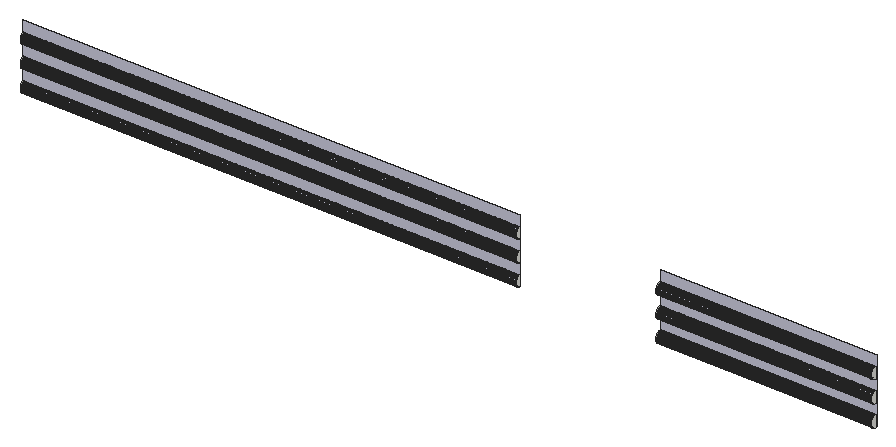
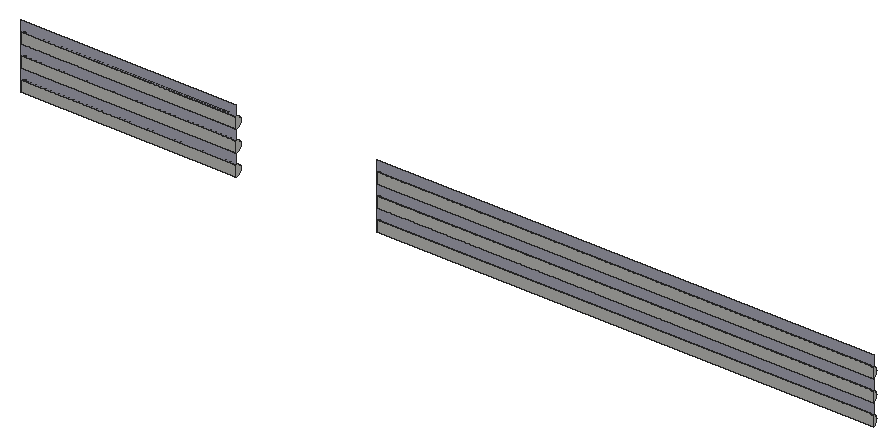
# SketchUp Ruby script. Lengths in millimetres.
U = 1.mm
M = Sketchup.active_model
def pt(a) = Geom::Point3d.new(a.map { |v| v * U })
def face(e, loops, mat)
  f = e.add_face(loops[0].map { |a| pt(a) })
  loops[1..].each { |l| e.add_face(l.map { |a| pt(a) }).erase! }
  f.material = f.back_material = mat if mat
  f
end
# faces: each face lists its corners as indices into pts; further lists are holes
def faces(e, pts, list, mat = nil) = list.each { |f| face(e, (f[0].is_a?(Array) ? f : [f]).map { |l| l.map { |i| pts[i] } }, mat) }
# xy, xz, yz: faces in a plane at the given z, y or x. An outline is a flat list of corners, or four numbers for a rectangle; further outlines are holes
def ring(l) = l.size == 4 ? [[l[0], l[1]], [l[2], l[1]], [l[2], l[3]], [l[0], l[3]]] : l.each_slice(2).to_a
def flat(e, list, mat, &to3) = list.each { |f| face(e, (f[0].is_a?(Array) ? f : [f]).map { |l| ring(l).map { |u, v| to3.(u, v) } }, mat) }
def xy(e, z, list, mat = nil) = flat(e, list, mat) { |x, y| [x, y, z] }
def xz(e, y, list, mat = nil) = flat(e, list, mat) { |x, z| [x, y, z] }
def yz(e, x, list, mat = nil) = flat(e, list, mat) { |y, z| [x, y, z] }
def lines(e, pts, list) = list.each { |a, b| e.add_line(pt(pts[a]), pt(pts[b])) }
# prism: a flat outline (further loops are holes) pulled along v
def prism(e, loops, v, mat = nil)
  f = face(e, loops, mat); d = Geom::Vector3d.new(v.map { |x| x * U })
  f.pushpull(f.normal.samedirection?(d) ? d.length : -d.length)
end
def box(e, o, s, mat = nil) = prism(e, [[o, [o[0] + s[0], o[1], o[2]], [o[0] + s[0], o[1] + s[1], o[2]], [o[0], o[1] + s[1], o[2]]]], [0, 0, s[2]], mat)
def at(x, y, z, deg = 0) = Geom::Transformation.translation(pt([x, y, z])) * Geom::Transformation.rotation(ORIGIN, Z_AXIS, deg.degrees)
def axes(o, x, y, z) = Geom::Transformation.new([*x, 0, *y, 0, *z, 0, *pt(o).to_a, 1])
def part(name) = M.definitions.add(name)
# library, detail: a bought-in or finely detailed component or shape, given as its bounding box
def library(name, o, s) = part(name).tap { |d| box(d.entities, o, s) }
def detail(e, o, s) = box(e.add_group.entities, o, s)
def put(e, d, t, mat = nil) = e.add_instance(d, t).tap { |i| i.material = mat if mat }
def group(e, t, mat = nil) = e.add_group.tap { |g| g.transformation = t; g.material = mat if mat }.entities
root = M.entities
M.materials.add("[0116_Lavender]").color = [197, 197, 214]
xz(root,16548.1,[[11038.5,11141.1,25059.3,11445.9],[29021.7,11141.1,35117.7,11445.9],[11038.5,11750.7,25059.3,12055.5],[29021.7,11750.7,35117.7,12055.5],[11038.5,12360.3,25059.3,12665.1],
  [29021.7,12360.3,35117.7,12665.1]])
xz(root,16548.1,[[11038.5,11445.9,25059.3,11750.7],[29021.7,11445.9,35117.7,11750.7],[11038.5,12055.5,25059.3,12360.3],[29021.7,12055.5,35117.7,12360.3],[11038.5,12665.1,25059.3,12969.9],
  [29021.7,12665.1,35117.7,12969.9]],"[0116_Lavender]")
yz(root,11038.5,[[16548.1,11141.1,16536.2,11146.4,16524.8,11152.7,16514,11159.8,16503.7,11167.8,16494.1,11176.6,16485.2,11186.1,16477.1,11196.2,16469.8,11207,16463.4,11218.3,16458,11230.1,16453.4,11242.3,16449.9,11254.8,16447.3,11267.6,16445.8,11280.5,16445.3,11293.5,16445.8,11306.5,16447.3,11319.4,16449.9,11332.1,16453.4,11344.6,16458,11356.8,16463.4,11368.6,16469.8,11379.9,16477.1,11390.7,16485.2,11400.9,16494.1,11410.4,16503.7,11419.2,16514,11427.1,16524.8,11434.3,16536.2,11440.5,16548.1,11445.9],[16548.1,11750.7,16536.2,11756,16524.8,11762.3,16514,11769.4,16503.7,11777.4,16494.1,11786.2,16485.2,11795.7,16477.1,11805.8,16469.8,11816.6,16463.4,11827.9,16458,11839.7,16453.4,11851.9,16449.9,11864.4,16447.3,11877.2,16445.8,11890.1,16445.3,11903.1,16445.8,11916.1,16447.3,11929,16449.9,11941.7,16453.4,11954.2,16458,11966.4,16463.4,11978.2,16469.8,11989.5,16477.1,12000.3,16485.2,12010.5,16494.1,12020,16503.7,12028.8,16514,12036.7,16524.8,12043.9,16536.2,12050.1,16548.1,12055.5],[16548.1,12360.3,16536.2,12365.6,16524.8,12371.9,16514,12379,16503.7,12387,16494.1,12395.8,16485.2,12405.3,16477.1,12415.4,16469.8,12426.2,16463.4,12437.5,16458,12449.3,16453.4,12461.5,16449.9,12474,16447.3,12486.8,16445.8,12499.7,16445.3,12512.7,16445.8,12525.7,16447.3,12538.6,16449.9,12551.3,16453.4,12563.8,16458,12576,16463.4,12587.8,16469.8,12599.1,16477.1,12609.9,16485.2,12620.1,16494.1,12629.6,16503.7,12638.4,16514,12646.3,16524.8,12653.5,16536.2,12659.7,16548.1,12665.1]])
yz(root,25059.3,[[16548.1,11141.1,16548.1,11445.9,16536.2,11440.5,16524.8,11434.3,16514,11427.1,16503.7,11419.2,16494.1,11410.4,16485.2,11400.9,16477.1,11390.7,16469.8,11379.9,16463.4,11368.6,16458,11356.8,16453.4,11344.6,16449.9,11332.1,16447.3,11319.4,16445.8,11306.5,16445.3,11293.5,16445.8,11280.5,16447.3,11267.6,16449.9,11254.8,16453.4,11242.3,16458,11230.1,16463.4,11218.3,16469.8,11207,16477.1,11196.2,16485.2,11186.1,16494.1,11176.6,16503.7,11167.8,16514,11159.8,16524.8,11152.7,16536.2,11146.4],[16548.1,11750.7,16548.1,12055.5,16536.2,12050.1,16524.8,12043.9,16514,12036.7,16503.7,12028.8,16494.1,12020,16485.2,12010.5,16477.1,12000.3,16469.8,11989.5,16463.4,11978.2,16458,11966.4,16453.4,11954.2,16449.9,11941.7,16447.3,11929,16445.8,11916.1,16445.3,11903.1,16445.8,11890.1,16447.3,11877.2,16449.9,11864.4,16453.4,11851.9,16458,11839.7,16463.4,11827.9,16469.8,11816.6,16477.1,11805.8,16485.2,11795.7,16494.1,11786.2,16503.7,11777.4,16514,11769.4,16524.8,11762.3,16536.2,11756],[16548.1,12360.3,16548.1,12665.1,16536.2,12659.7,16524.8,12653.5,16514,12646.3,16503.7,12638.4,16494.1,12629.6,16485.2,12620.1,16477.1,12609.9,16469.8,12599.1,16463.4,12587.8,16458,12576,16453.4,12563.8,16449.9,12551.3,16447.3,12538.6,16445.8,12525.7,16445.3,12512.7,16445.8,12499.7,16447.3,12486.8,16449.9,12474,16453.4,12461.5,16458,12449.3,16463.4,12437.5,16469.8,12426.2,16477.1,12415.4,16485.2,12405.3,16494.1,12395.8,16503.7,12387,16514,12379,16524.8,12371.9,16536.2,12365.6]])
yz(root,29021.7,[[16548.1,11141.1,16540.1,11141.3,16532.2,11141.9,16524.3,11143,16516.4,11144.4,16508.7,11146.3,16501,11148.5,16493.5,11151.2,16486.1,11154.3,16478.9,11157.7,16471.9,11161.5,16465.1,11165.7,16458.5,11170.2,16452.2,11175,16446.1,11180.2,16440.3,11185.7,16434.8,11191.5,16429.7,11197.6,16424.8,11203.9,16420.3,11210.5,16416.1,11217.3,16412.3,11224.3,16408.9,11231.5,16405.8,11238.9,16403.2,11246.4,16400.9,11254,16399,11261.8,16397.6,11269.6,16396.5,11277.5,16395.9,11285.5,16395.7,11293.5,16395.9,11301.5,16396.5,11309.4,16397.6,11317.3,16399,11325.2,16400.9,11332.9,16403.2,11340.6,16405.8,11348.1,16408.9,11355.5,16412.3,11362.7,16416.1,11369.7,16420.3,11376.5,16424.8,11383.1,16429.7,11389.4,16434.8,11395.5,16440.3,11401.2,16446.1,11406.7,16452.2,11411.9,16458.5,11416.8,16465.1,11421.3,16471.9,11425.5,16478.9,11429.3,16486.1,11432.7,16493.5,11435.8,16501,11438.4,16508.7,11440.7,16516.4,11442.5,16524.3,11444,16532.2,11445,16540.1,11445.7,16548.1,11445.9],[16548.1,11750.7,16540.1,11750.9,16532.2,11751.5,16524.3,11752.6,16516.4,11754,16508.7,11755.9,16501,11758.1,16493.5,11760.8,16486.1,11763.9,16478.9,11767.3,16471.9,11771.1,16465.1,11775.3,16458.5,11779.8,16452.2,11784.6,16446.1,11789.8,16440.3,11795.3,16434.8,11801.1,16429.7,11807.2,16424.8,11813.5,16420.3,11820.1,16416.1,11826.9,16412.3,11833.9,16408.9,11841.1,16405.8,11848.5,16403.2,11856,16400.9,11863.6,16399,11871.4,16397.6,11879.2,16396.5,11887.1,16395.9,11895.1,16395.7,11903.1,16395.9,11911.1,16396.5,11919,16397.6,11926.9,16399,11934.8,16400.9,11942.5,16403.2,11950.2,16405.8,11957.7,16408.9,11965.1,16412.3,11972.3,16416.1,11979.3,16420.3,11986.1,16424.8,11992.7,16429.7,11999,16434.8,12005.1,16440.3,12010.8,16446.1,12016.3,16452.2,12021.5,16458.5,12026.4,16465.1,12030.9,16471.9,12035.1,16478.9,12038.9,16486.1,12042.3,16493.5,12045.4,16501,12048,16508.7,12050.3,16516.4,12052.1,16524.3,12053.6,16532.2,12054.6,16540.1,12055.3,16548.1,12055.5],[16548.1,12360.3,16540.1,12360.5,16532.2,12361.1,16524.3,12362.2,16516.4,12363.6,16508.7,12365.5,16501,12367.7,16493.5,12370.4,16486.1,12373.5,16478.9,12376.9,16471.9,12380.7,16465.1,12384.9,16458.5,12389.4,16452.2,12394.2,16446.1,12399.4,16440.3,12404.9,16434.8,12410.7,16429.7,12416.8,16424.8,12423.1,16420.3,12429.7,16416.1,12436.5,16412.3,12443.5,16408.9,12450.7,16405.8,12458.1,16403.2,12465.6,16400.9,12473.2,16399,12481,16397.6,12488.8,16396.5,12496.7,16395.9,12504.7,16395.7,12512.7,16395.9,12520.7,16396.5,12528.6,16397.6,12536.5,16399,12544.4,16400.9,12552.1,16403.2,12559.8,16405.8,12567.3,16408.9,12574.7,16412.3,12581.9,16416.1,12588.9,16420.3,12595.7,16424.8,12602.3,16429.7,12608.6,16434.8,12614.7,16440.3,12620.4,16446.1,12625.9,16452.2,12631.1,16458.5,12636,16465.1,12640.5,16471.9,12644.7,16478.9,12648.5,16486.1,12651.9,16493.5,12655,16501,12657.6,16508.7,12659.9,16516.4,12661.7,16524.3,12663.2,16532.2,12664.2,16540.1,12664.9,16548.1,12665.1]])
yz(root,35117.7,[[16548.1,11141.1,16548.1,11445.9,16540.1,11445.7,16532.2,11445,16524.3,11444,16516.4,11442.5,16508.7,11440.7,16501,11438.4,16493.5,11435.8,16486.1,11432.7,16478.9,11429.3,16471.9,11425.5,16465.1,11421.3,16458.5,11416.8,16452.2,11411.9,16446.1,11406.7,16440.3,11401.2,16434.8,11395.5,16429.7,11389.4,16424.8,11383.1,16420.3,11376.5,16416.1,11369.7,16412.3,11362.7,16408.9,11355.5,16405.8,11348.1,16403.2,11340.6,16400.9,11332.9,16399,11325.2,16397.6,11317.3,16396.5,11309.4,16395.9,11301.5,16395.7,11293.5,16395.9,11285.5,16396.5,11277.5,16397.6,11269.6,16399,11261.8,16400.9,11254,16403.2,11246.4,16405.8,11238.9,16408.9,11231.5,16412.3,11224.3,16416.1,11217.3,16420.3,11210.5,16424.8,11203.9,16429.7,11197.6,16434.8,11191.5,16440.3,11185.7,16446.1,11180.2,16452.2,11175,16458.5,11170.2,16465.1,11165.7,16471.9,11161.5,16478.9,11157.7,16486.1,11154.3,16493.5,11151.2,16501,11148.5,16508.7,11146.3,16516.4,11144.4,16524.3,11143,16532.2,11141.9,16540.1,11141.3],[16548.1,11750.7,16548.1,12055.5,16540.1,12055.3,16532.2,12054.6,16524.3,12053.6,16516.4,12052.1,16508.7,12050.3,16501,12048,16493.5,12045.4,16486.1,12042.3,16478.9,12038.9,16471.9,12035.1,16465.1,12030.9,16458.5,12026.4,16452.2,12021.5,16446.1,12016.3,16440.3,12010.8,16434.8,12005.1,16429.7,11999,16424.8,11992.7,16420.3,11986.1,16416.1,11979.3,16412.3,11972.3,16408.9,11965.1,16405.8,11957.7,16403.2,11950.2,16400.9,11942.5,16399,11934.8,16397.6,11926.9,16396.5,11919,16395.9,11911.1,16395.7,11903.1,16395.9,11895.1,16396.5,11887.1,16397.6,11879.2,16399,11871.4,16400.9,11863.6,16403.2,11856,16405.8,11848.5,16408.9,11841.1,16412.3,11833.9,16416.1,11826.9,16420.3,11820.1,16424.8,11813.5,16429.7,11807.2,16434.8,11801.1,16440.3,11795.3,16446.1,11789.8,16452.2,11784.6,16458.5,11779.8,16465.1,11775.3,16471.9,11771.1,16478.9,11767.3,16486.1,11763.9,16493.5,11760.8,16501,11758.1,16508.7,11755.9,16516.4,11754,16524.3,11752.6,16532.2,11751.5,16540.1,11750.9],[16548.1,12360.3,16548.1,12665.1,16540.1,12664.9,16532.2,12664.2,16524.3,12663.2,16516.4,12661.7,16508.7,12659.9,16501,12657.6,16493.5,12655,16486.1,12651.9,16478.9,12648.5,16471.9,12644.7,16465.1,12640.5,16458.5,12636,16452.2,12631.1,16446.1,12625.9,16440.3,12620.4,16434.8,12614.7,16429.7,12608.6,16424.8,12602.3,16420.3,12595.7,16416.1,12588.9,16412.3,12581.9,16408.9,12574.7,16405.8,12567.3,16403.2,12559.8,16400.9,12552.1,16399,12544.4,16397.6,12536.5,16396.5,12528.6,16395.9,12520.7,16395.7,12512.7,16395.9,12504.7,16396.5,12496.7,16397.6,12488.8,16399,12481,16400.9,12473.2,16403.2,12465.6,16405.8,12458.1,16408.9,12450.7,16412.3,12443.5,16416.1,12436.5,16420.3,12429.7,16424.8,12423.1,16429.7,12416.8,16434.8,12410.7,16440.3,12404.9,16446.1,12399.4,16452.2,12394.2,16458.5,12389.4,16465.1,12384.9,16471.9,12380.7,16478.9,12376.9,16486.1,12373.5,16493.5,12370.4,16501,12367.7,16508.7,12365.5,16516.4,12363.6,16524.3,12362.2,16532.2,12361.1,16540.1,12360.5]])
p = [[25059.3,16548.1,11141.1],[25059.3,16536.2,11146.4],[11038.5,16536.2,11146.4],[11038.5,16548.1,11141.1],[35117.7,16548.1,11141.1],[35117.7,16540.1,11141.3],
  [29021.7,16540.1,11141.3],[29021.7,16548.1,11141.1],[35117.7,16532.2,11141.9],[29021.7,16532.2,11141.9],[35117.7,16524.3,11143],[29021.7,16524.3,11143],
  [35117.7,16516.4,11144.4],[29021.7,16516.4,11144.4],[35117.7,16508.7,11146.3],[29021.7,16508.7,11146.3],[35117.7,16501,11148.5],[29021.7,16501,11148.5],
  [25059.3,16524.8,11152.7],[11038.5,16524.8,11152.7],[35117.7,16493.5,11151.2],[29021.7,16493.5,11151.2],[35117.7,16486.1,11154.3],[29021.7,16486.1,11154.3],
  [25059.3,16514,11159.8],[11038.5,16514,11159.8],[35117.7,16478.9,11157.7],[29021.7,16478.9,11157.7],[35117.7,16471.9,11161.5],[29021.7,16471.9,11161.5],
  [25059.3,16503.7,11167.8],[11038.5,16503.7,11167.8],[35117.7,16465.1,11165.7],[29021.7,16465.1,11165.7],[35117.7,16458.5,11170.2],[29021.7,16458.5,11170.2],
  [25059.3,16494.1,11176.6],[11038.5,16494.1,11176.6],[35117.7,16452.2,11175],[29021.7,16452.2,11175],[35117.7,16446.1,11180.2],[29021.7,16446.1,11180.2],
  [25059.3,16485.2,11186.1],[11038.5,16485.2,11186.1],[35117.7,16440.3,11185.7],[29021.7,16440.3,11185.7],[35117.7,16434.8,11191.5],[29021.7,16434.8,11191.5],
  [25059.3,16477.1,11196.2],[11038.5,16477.1,11196.2],[35117.7,16429.7,11197.6],[29021.7,16429.7,11197.6],[25059.3,16469.8,11207],[11038.5,16469.8,11207],
  [35117.7,16424.8,11203.9],[29021.7,16424.8,11203.9],[35117.7,16420.3,11210.5],[29021.7,16420.3,11210.5],[25059.3,16463.4,11218.3],[11038.5,16463.4,11218.3],
  [35117.7,16416.1,11217.3],[29021.7,16416.1,11217.3],[35117.7,16412.3,11224.3],[29021.7,16412.3,11224.3],[25059.3,16458,11230.1],[11038.5,16458,11230.1],
  [35117.7,16408.9,11231.5],[29021.7,16408.9,11231.5],[25059.3,16453.4,11242.3],[11038.5,16453.4,11242.3],[35117.7,16405.8,11238.9],[29021.7,16405.8,11238.9],
  [35117.7,16403.2,11246.4],[29021.7,16403.2,11246.4],[25059.3,16449.9,11254.8],[11038.5,16449.9,11254.8],[35117.7,16400.9,11254],[29021.7,16400.9,11254],
  [35117.7,16399,11261.8],[29021.7,16399,11261.8],[25059.3,16447.3,11267.6],[11038.5,16447.3,11267.6],[35117.7,16397.6,11269.6],[29021.7,16397.6,11269.6],
  [25059.3,16445.8,11280.5],[11038.5,16445.8,11280.5],[35117.7,16396.5,11277.5],[29021.7,16396.5,11277.5],[35117.7,16395.9,11285.5],[29021.7,16395.9,11285.5],
  [25059.3,16445.3,11293.5],[11038.5,16445.3,11293.5],[35117.7,16395.7,11293.5],[29021.7,16395.7,11293.5],[35117.7,16395.9,11301.5],[29021.7,16395.9,11301.5],
  [25059.3,16445.8,11306.5],[11038.5,16445.8,11306.5],[35117.7,16396.5,11309.4],[29021.7,16396.5,11309.4],[25059.3,16447.3,11319.4],[11038.5,16447.3,11319.4],
  [35117.7,16397.6,11317.3],[29021.7,16397.6,11317.3],[35117.7,16399,11325.2],[29021.7,16399,11325.2],[25059.3,16449.9,11332.1],[11038.5,16449.9,11332.1],
  [35117.7,16400.9,11332.9],[29021.7,16400.9,11332.9],[25059.3,16453.4,11344.6],[11038.5,16453.4,11344.6],[35117.7,16403.2,11340.6],[29021.7,16403.2,11340.6],
  [35117.7,16405.8,11348.1],[29021.7,16405.8,11348.1],[25059.3,16458,11356.8],[11038.5,16458,11356.8],[35117.7,16408.9,11355.5],[29021.7,16408.9,11355.5],
  [35117.7,16412.3,11362.7],[29021.7,16412.3,11362.7],[25059.3,16463.4,11368.6],[11038.5,16463.4,11368.6],[35117.7,16416.1,11369.7],[29021.7,16416.1,11369.7],
  [25059.3,16469.8,11379.9],[11038.5,16469.8,11379.9],[35117.7,16420.3,11376.5],[29021.7,16420.3,11376.5],[35117.7,16424.8,11383.1],[29021.7,16424.8,11383.1],
  [25059.3,16477.1,11390.7],[11038.5,16477.1,11390.7],[35117.7,16429.7,11389.4],[29021.7,16429.7,11389.4],[35117.7,16434.8,11395.5],[29021.7,16434.8,11395.5],
  [25059.3,16485.2,11400.9],[11038.5,16485.2,11400.9],[35117.7,16440.3,11401.2],[29021.7,16440.3,11401.2],[25059.3,16494.1,11410.4],[11038.5,16494.1,11410.4],
  [35117.7,16446.1,11406.7],[29021.7,16446.1,11406.7],[35117.7,16452.2,11411.9],[29021.7,16452.2,11411.9],[25059.3,16503.7,11419.2],[11038.5,16503.7,11419.2],
  [35117.7,16458.5,11416.8],[29021.7,16458.5,11416.8],[35117.7,16465.1,11421.3],[29021.7,16465.1,11421.3],[25059.3,16514,11427.1],[11038.5,16514,11427.1],
  [35117.7,16471.9,11425.5],[29021.7,16471.9,11425.5],[35117.7,16478.9,11429.3],[29021.7,16478.9,11429.3],[25059.3,16524.8,11434.3],[11038.5,16524.8,11434.3],
  [35117.7,16486.1,11432.7],[29021.7,16486.1,11432.7],[35117.7,16493.5,11435.8],[29021.7,16493.5,11435.8],[25059.3,16536.2,11440.5],[11038.5,16536.2,11440.5],
  [35117.7,16501,11438.4],[29021.7,16501,11438.4],[35117.7,16508.7,11440.7],[29021.7,16508.7,11440.7],[25059.3,16548.1,11445.9],[11038.5,16548.1,11445.9],
  [35117.7,16516.4,11442.5],[29021.7,16516.4,11442.5],[35117.7,16524.3,11444],[29021.7,16524.3,11444],[35117.7,16532.2,11445],[29021.7,16532.2,11445],
  [35117.7,16540.1,11445.7],[29021.7,16540.1,11445.7],[35117.7,16548.1,11445.9],[29021.7,16548.1,11445.9],[25059.3,16548.1,11750.7],[25059.3,16536.2,11756],
  [11038.5,16536.2,11756],[11038.5,16548.1,11750.7],[35117.7,16548.1,11750.7],[35117.7,16540.1,11750.9],[29021.7,16540.1,11750.9],[29021.7,16548.1,11750.7],
  [35117.7,16532.2,11751.5],[29021.7,16532.2,11751.5],[35117.7,16524.3,11752.6],[29021.7,16524.3,11752.6],[35117.7,16516.4,11754],[29021.7,16516.4,11754],
  [35117.7,16508.7,11755.9],[29021.7,16508.7,11755.9],[35117.7,16501,11758.1],[29021.7,16501,11758.1],[25059.3,16524.8,11762.3],[11038.5,16524.8,11762.3],
  [35117.7,16493.5,11760.8],[29021.7,16493.5,11760.8],[35117.7,16486.1,11763.9],[29021.7,16486.1,11763.9],[25059.3,16514,11769.4],[11038.5,16514,11769.4],
  [35117.7,16478.9,11767.3],[29021.7,16478.9,11767.3],[35117.7,16471.9,11771.1],[29021.7,16471.9,11771.1],[25059.3,16503.7,11777.4],[11038.5,16503.7,11777.4],
  [35117.7,16465.1,11775.3],[29021.7,16465.1,11775.3],[35117.7,16458.5,11779.8],[29021.7,16458.5,11779.8],[25059.3,16494.1,11786.2],[11038.5,16494.1,11786.2],
  [35117.7,16452.2,11784.6],[29021.7,16452.2,11784.6],[35117.7,16446.1,11789.8],[29021.7,16446.1,11789.8],[25059.3,16485.2,11795.7],[11038.5,16485.2,11795.7],
  [35117.7,16440.3,11795.3],[29021.7,16440.3,11795.3],[35117.7,16434.8,11801.1],[29021.7,16434.8,11801.1],[25059.3,16477.1,11805.8],[11038.5,16477.1,11805.8],
  [35117.7,16429.7,11807.2],[29021.7,16429.7,11807.2],[25059.3,16469.8,11816.6],[11038.5,16469.8,11816.6],[35117.7,16424.8,11813.5],[29021.7,16424.8,11813.5],
  [35117.7,16420.3,11820.1],[29021.7,16420.3,11820.1],[25059.3,16463.4,11827.9],[11038.5,16463.4,11827.9],[35117.7,16416.1,11826.9],[29021.7,16416.1,11826.9],
  [35117.7,16412.3,11833.9],[29021.7,16412.3,11833.9],[25059.3,16458,11839.7],[11038.5,16458,11839.7],[35117.7,16408.9,11841.1],[29021.7,16408.9,11841.1],
  [25059.3,16453.4,11851.9],[11038.5,16453.4,11851.9],[35117.7,16405.8,11848.5],[29021.7,16405.8,11848.5],[35117.7,16403.2,11856],[29021.7,16403.2,11856],
  [25059.3,16449.9,11864.4],[11038.5,16449.9,11864.4],[35117.7,16400.9,11863.6],[29021.7,16400.9,11863.6],[35117.7,16399,11871.4],[29021.7,16399,11871.4],
  [25059.3,16447.3,11877.2],[11038.5,16447.3,11877.2],[35117.7,16397.6,11879.2],[29021.7,16397.6,11879.2],[25059.3,16445.8,11890.1],[11038.5,16445.8,11890.1],
  [35117.7,16396.5,11887.1],[29021.7,16396.5,11887.1],[35117.7,16395.9,11895.1],[29021.7,16395.9,11895.1],[25059.3,16445.3,11903.1],[11038.5,16445.3,11903.1],
  [35117.7,16395.7,11903.1],[29021.7,16395.7,11903.1],[35117.7,16395.9,11911.1],[29021.7,16395.9,11911.1],[25059.3,16445.8,11916.1],[11038.5,16445.8,11916.1],
  [35117.7,16396.5,11919],[29021.7,16396.5,11919],[25059.3,16447.3,11929],[11038.5,16447.3,11929],[35117.7,16397.6,11926.9],[29021.7,16397.6,11926.9],
  [35117.7,16399,11934.8],[29021.7,16399,11934.8],[25059.3,16449.9,11941.7],[11038.5,16449.9,11941.7],[35117.7,16400.9,11942.5],[29021.7,16400.9,11942.5],
  [25059.3,16453.4,11954.2],[11038.5,16453.4,11954.2],[35117.7,16403.2,11950.2],[29021.7,16403.2,11950.2],[35117.7,16405.8,11957.7],[29021.7,16405.8,11957.7],
  [25059.3,16458,11966.4],[11038.5,16458,11966.4],[35117.7,16408.9,11965.1],[29021.7,16408.9,11965.1],[35117.7,16412.3,11972.3],[29021.7,16412.3,11972.3],
  [25059.3,16463.4,11978.2],[11038.5,16463.4,11978.2],[35117.7,16416.1,11979.3],[29021.7,16416.1,11979.3],[25059.3,16469.8,11989.5],[11038.5,16469.8,11989.5],
  [35117.7,16420.3,11986.1],[29021.7,16420.3,11986.1],[35117.7,16424.8,11992.7],[29021.7,16424.8,11992.7],[25059.3,16477.1,12000.3],[11038.5,16477.1,12000.3],
  [35117.7,16429.7,11999],[29021.7,16429.7,11999],[35117.7,16434.8,12005.1],[29021.7,16434.8,12005.1],[25059.3,16485.2,12010.5],[11038.5,16485.2,12010.5],
  [35117.7,16440.3,12010.8],[29021.7,16440.3,12010.8],[25059.3,16494.1,12020],[11038.5,16494.1,12020],[35117.7,16446.1,12016.3],[29021.7,16446.1,12016.3],
  [35117.7,16452.2,12021.5],[29021.7,16452.2,12021.5],[25059.3,16503.7,12028.8],[11038.5,16503.7,12028.8],[35117.7,16458.5,12026.4],[29021.7,16458.5,12026.4],
  [35117.7,16465.1,12030.9],[29021.7,16465.1,12030.9],[25059.3,16514,12036.7],[11038.5,16514,12036.7],[35117.7,16471.9,12035.1],[29021.7,16471.9,12035.1],
  [35117.7,16478.9,12038.9],[29021.7,16478.9,12038.9],[25059.3,16524.8,12043.9],[11038.5,16524.8,12043.9],[35117.7,16486.1,12042.3],[29021.7,16486.1,12042.3],
  [35117.7,16493.5,12045.4],[29021.7,16493.5,12045.4],[25059.3,16536.2,12050.1],[11038.5,16536.2,12050.1],[35117.7,16501,12048],[29021.7,16501,12048],
  [35117.7,16508.7,12050.3],[29021.7,16508.7,12050.3],[25059.3,16548.1,12055.5],[11038.5,16548.1,12055.5],[35117.7,16516.4,12052.1],[29021.7,16516.4,12052.1],
  [35117.7,16524.3,12053.6],[29021.7,16524.3,12053.6],[35117.7,16532.2,12054.6],[29021.7,16532.2,12054.6],[35117.7,16540.1,12055.3],[29021.7,16540.1,12055.3],
  [35117.7,16548.1,12055.5],[29021.7,16548.1,12055.5],[25059.3,16548.1,12360.3],[25059.3,16536.2,12365.6],[11038.5,16536.2,12365.6],[11038.5,16548.1,12360.3],
  [35117.7,16548.1,12360.3],[35117.7,16540.1,12360.5],[29021.7,16540.1,12360.5],[29021.7,16548.1,12360.3],[35117.7,16532.2,12361.1],[29021.7,16532.2,12361.1],
  [35117.7,16524.3,12362.2],[29021.7,16524.3,12362.2],[35117.7,16516.4,12363.6],[29021.7,16516.4,12363.6],[35117.7,16508.7,12365.5],[29021.7,16508.7,12365.5],
  [35117.7,16501,12367.7],[29021.7,16501,12367.7],[25059.3,16524.8,12371.9],[11038.5,16524.8,12371.9],[35117.7,16493.5,12370.4],[29021.7,16493.5,12370.4],
  [35117.7,16486.1,12373.5],[29021.7,16486.1,12373.5],[25059.3,16514,12379],[11038.5,16514,12379],[35117.7,16478.9,12376.9],[29021.7,16478.9,12376.9],
  [35117.7,16471.9,12380.7],[29021.7,16471.9,12380.7],[25059.3,16503.7,12387],[11038.5,16503.7,12387],[35117.7,16465.1,12384.9],[29021.7,16465.1,12384.9],
  [35117.7,16458.5,12389.4],[29021.7,16458.5,12389.4],[25059.3,16494.1,12395.8],[11038.5,16494.1,12395.8],[35117.7,16452.2,12394.2],[29021.7,16452.2,12394.2],
  [35117.7,16446.1,12399.4],[29021.7,16446.1,12399.4],[25059.3,16485.2,12405.3],[11038.5,16485.2,12405.3],[35117.7,16440.3,12404.9],[29021.7,16440.3,12404.9],
  [35117.7,16434.8,12410.7],[29021.7,16434.8,12410.7],[25059.3,16477.1,12415.4],[11038.5,16477.1,12415.4],[35117.7,16429.7,12416.8],[29021.7,16429.7,12416.8],
  [25059.3,16469.8,12426.2],[11038.5,16469.8,12426.2],[35117.7,16424.8,12423.1],[29021.7,16424.8,12423.1],[35117.7,16420.3,12429.7],[29021.7,16420.3,12429.7],
  [25059.3,16463.4,12437.5],[11038.5,16463.4,12437.5],[35117.7,16416.1,12436.5],[29021.7,16416.1,12436.5],[35117.7,16412.3,12443.5],[29021.7,16412.3,12443.5],
  [25059.3,16458,12449.3],[11038.5,16458,12449.3],[35117.7,16408.9,12450.7],[29021.7,16408.9,12450.7],[25059.3,16453.4,12461.5],[11038.5,16453.4,12461.5],
  [35117.7,16405.8,12458.1],[29021.7,16405.8,12458.1],[35117.7,16403.2,12465.6],[29021.7,16403.2,12465.6],[25059.3,16449.9,12474],[11038.5,16449.9,12474],
  [35117.7,16400.9,12473.2],[29021.7,16400.9,12473.2],[35117.7,16399,12481],[29021.7,16399,12481],[25059.3,16447.3,12486.8],[11038.5,16447.3,12486.8],
  [35117.7,16397.6,12488.8],[29021.7,16397.6,12488.8],[25059.3,16445.8,12499.7],[11038.5,16445.8,12499.7],[35117.7,16396.5,12496.7],[29021.7,16396.5,12496.7],
  [35117.7,16395.9,12504.7],[29021.7,16395.9,12504.7],[25059.3,16445.3,12512.7],[11038.5,16445.3,12512.7],[35117.7,16395.7,12512.7],[29021.7,16395.7,12512.7],
  [35117.7,16395.9,12520.7],[29021.7,16395.9,12520.7],[25059.3,16445.8,12525.7],[11038.5,16445.8,12525.7],[35117.7,16396.5,12528.6],[29021.7,16396.5,12528.6],
  [25059.3,16447.3,12538.6],[11038.5,16447.3,12538.6],[35117.7,16397.6,12536.5],[29021.7,16397.6,12536.5],[35117.7,16399,12544.4],[29021.7,16399,12544.4],
  [25059.3,16449.9,12551.3],[11038.5,16449.9,12551.3],[35117.7,16400.9,12552.1],[29021.7,16400.9,12552.1],[25059.3,16453.4,12563.8],[11038.5,16453.4,12563.8],
  [35117.7,16403.2,12559.8],[29021.7,16403.2,12559.8],[35117.7,16405.8,12567.3],[29021.7,16405.8,12567.3],[25059.3,16458,12576],[11038.5,16458,12576],
  [35117.7,16408.9,12574.7],[29021.7,16408.9,12574.7],[35117.7,16412.3,12581.9],[29021.7,16412.3,12581.9],[25059.3,16463.4,12587.8],[11038.5,16463.4,12587.8],
  [35117.7,16416.1,12588.9],[29021.7,16416.1,12588.9],[25059.3,16469.8,12599.1],[11038.5,16469.8,12599.1],[35117.7,16420.3,12595.7],[29021.7,16420.3,12595.7],
  [35117.7,16424.8,12602.3],[29021.7,16424.8,12602.3],[25059.3,16477.1,12609.9],[11038.5,16477.1,12609.9],[35117.7,16429.7,12608.6],[29021.7,16429.7,12608.6],
  [35117.7,16434.8,12614.7],[29021.7,16434.8,12614.7],[25059.3,16485.2,12620.1],[11038.5,16485.2,12620.1],[35117.7,16440.3,12620.4],[29021.7,16440.3,12620.4],
  [25059.3,16494.1,12629.6],[11038.5,16494.1,12629.6],[35117.7,16446.1,12625.9],[29021.7,16446.1,12625.9],[35117.7,16452.2,12631.1],[29021.7,16452.2,12631.1],
  [25059.3,16503.7,12638.4],[11038.5,16503.7,12638.4],[35117.7,16458.5,12636],[29021.7,16458.5,12636],[35117.7,16465.1,12640.5],[29021.7,16465.1,12640.5],
  [25059.3,16514,12646.3],[11038.5,16514,12646.3],[35117.7,16471.9,12644.7],[29021.7,16471.9,12644.7],[35117.7,16478.9,12648.5],[29021.7,16478.9,12648.5],
  [25059.3,16524.8,12653.5],[11038.5,16524.8,12653.5],[35117.7,16486.1,12651.9],[29021.7,16486.1,12651.9],[35117.7,16493.5,12655],[29021.7,16493.5,12655],
  [25059.3,16536.2,12659.7],[11038.5,16536.2,12659.7],[35117.7,16501,12657.6],[29021.7,16501,12657.6],[35117.7,16508.7,12659.9],[29021.7,16508.7,12659.9],
  [25059.3,16548.1,12665.1],[11038.5,16548.1,12665.1],[35117.7,16516.4,12661.7],[29021.7,16516.4,12661.7],[35117.7,16524.3,12663.2],[29021.7,16524.3,12663.2],
  [35117.7,16532.2,12664.2],[29021.7,16532.2,12664.2],[35117.7,16540.1,12664.9],[29021.7,16540.1,12664.9],[35117.7,16548.1,12665.1],[29021.7,16548.1,12665.1]]
faces(root,p,[[0,1,2,3],[4,5,6,7],[5,8,9,6],[8,10,11,9],[10,12,13,11],[12,14,15,13],[14,16,17,15],[1,18,19,2],
  [16,20,21,17],[20,22,23,21],[18,24,25,19],[22,26,27,23],[26,28,29,27],[24,30,31,25],[28,32,33,29],[32,34,35,33],
  [30,36,37,31],[34,38,39,35],[38,40,41,39],[36,42,43,37],[40,44,45,41],[44,46,47,45],[42,48,49,43],[46,50,51,47],
  [48,52,53,49],[50,54,55,51],[54,56,57,55],[52,58,59,53],[56,60,61,57],[60,62,63,61],[58,64,65,59],[62,66,67,63],
  [64,68,69,65],[66,70,71,67],[70,72,73,71],[68,74,75,69],[72,76,77,73],[76,78,79,77],[74,80,81,75],[78,82,83,79],
  [80,84,85,81],[82,86,87,83],[86,88,89,87],[84,90,91,85],[88,92,93,89],[92,94,95,93],[90,96,97,91],[94,98,99,95],
  [96,100,101,97],[98,102,103,99],[102,104,105,103],[100,106,107,101],[104,108,109,105],[106,110,111,107],[108,112,113,109],[112,114,115,113],
  [110,116,117,111],[114,118,119,115],[118,120,121,119],[116,122,123,117],[120,124,125,121],[122,126,127,123],[124,128,129,125],[128,130,131,129],
  [126,132,133,127],[130,134,135,131],[134,136,137,135],[132,138,139,133],[136,140,141,137],[138,142,143,139],[140,144,145,141],[144,146,147,145],
  [142,148,149,143],[146,150,151,147],[150,152,153,151],[148,154,155,149],[152,156,157,153],[156,158,159,157],[154,160,161,155],[158,162,163,159],
  [162,164,165,163],[160,166,167,161],[164,168,169,165],[168,170,171,169],[166,172,173,167],[170,174,175,171],[174,176,177,175],[176,178,179,177],
  [178,180,181,179],[180,182,183,181],[184,185,186,187],[188,189,190,191],[189,192,193,190],[192,194,195,193],[194,196,197,195],[196,198,199,197],
  [198,200,201,199],[185,202,203,186],[200,204,205,201],[204,206,207,205],[202,208,209,203],[206,210,211,207],[210,212,213,211],[208,214,215,209],
  [212,216,217,213],[216,218,219,217],[214,220,221,215],[218,222,223,219],[222,224,225,223],[220,226,227,221],[224,228,229,225],[228,230,231,229],
  [226,232,233,227],[230,234,235,231],[232,236,237,233],[234,238,239,235],[238,240,241,239],[236,242,243,237],[240,244,245,241],[244,246,247,245],
  [242,248,249,243],[246,250,251,247],[248,252,253,249],[250,254,255,251],[254,256,257,255],[252,258,259,253],[256,260,261,257],[260,262,263,261],
  [258,264,265,259],[262,266,267,263],[264,268,269,265],[266,270,271,267],[270,272,273,271],[268,274,275,269],[272,276,277,273],[276,278,279,277],
  [274,280,281,275],[278,282,283,279],[280,284,285,281],[282,286,287,283],[286,288,289,287],[284,290,291,285],[288,292,293,289],[290,294,295,291],
  [292,296,297,293],[296,298,299,297],[294,300,301,295],[298,302,303,299],[302,304,305,303],[300,306,307,301],[304,308,309,305],[306,310,311,307],
  [308,312,313,309],[312,314,315,313],[310,316,317,311],[314,318,319,315],[318,320,321,319],[316,322,323,317],[320,324,325,321],[322,326,327,323],
  [324,328,329,325],[328,330,331,329],[326,332,333,327],[330,334,335,331],[334,336,337,335],[332,338,339,333],[336,340,341,337],[340,342,343,341],
  [338,344,345,339],[342,346,347,343],[346,348,349,347],[344,350,351,345],[348,352,353,349],[352,354,355,353],[350,356,357,351],[354,358,359,355],
  [358,360,361,359],[360,362,363,361],[362,364,365,363],[364,366,367,365],[368,369,370,371],[372,373,374,375],[373,376,377,374],[376,378,379,377],
  [378,380,381,379],[380,382,383,381],[382,384,385,383],[369,386,387,370],[384,388,389,385],[388,390,391,389],[386,392,393,387],[390,394,395,391],
  [394,396,397,395],[392,398,399,393],[396,400,401,397],[400,402,403,401],[398,404,405,399],[402,406,407,403],[406,408,409,407],[404,410,411,405],
  [408,412,413,409],[412,414,415,413],[410,416,417,411],[414,418,419,415],[416,420,421,417],[418,422,423,419],[422,424,425,423],[420,426,427,421],
  [424,428,429,425],[428,430,431,429],[426,432,433,427],[430,434,435,431],[432,436,437,433],[434,438,439,435],[438,440,441,439],[436,442,443,437],
  [440,444,445,441],[444,446,447,445],[442,448,449,443],[446,450,451,447],[448,452,453,449],[450,454,455,451],[454,456,457,455],[452,458,459,453],
  [456,460,461,457],[460,462,463,461],[458,464,465,459],[462,466,467,463],[464,468,469,465],[466,470,471,467],[470,472,473,471],[468,474,475,469],
  [472,476,477,473],[474,478,479,475],[476,480,481,477],[480,482,483,481],[478,484,485,479],[482,486,487,483],[486,488,489,487],[484,490,491,485],
  [488,492,493,489],[490,494,495,491],[492,496,497,493],[496,498,499,497],[494,500,501,495],[498,502,503,499],[502,504,505,503],[500,506,507,501],
  [504,508,509,505],[506,510,511,507],[508,512,513,509],[512,514,515,513],[510,516,517,511],[514,518,519,515],[518,520,521,519],[516,522,523,517],
  [520,524,525,521],[524,526,527,525],[522,528,529,523],[526,530,531,527],[530,532,533,531],[528,534,535,529],[532,536,537,533],[536,538,539,537],
  [534,540,541,535],[538,542,543,539],[542,544,545,543],[544,546,547,545],[546,548,549,547],[548,550,551,549]],"[0116_Lavender]")
